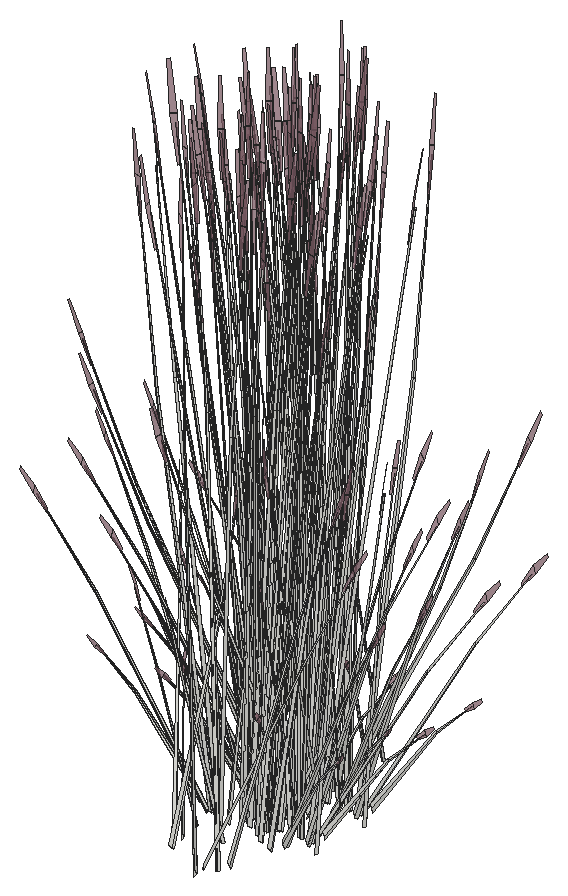
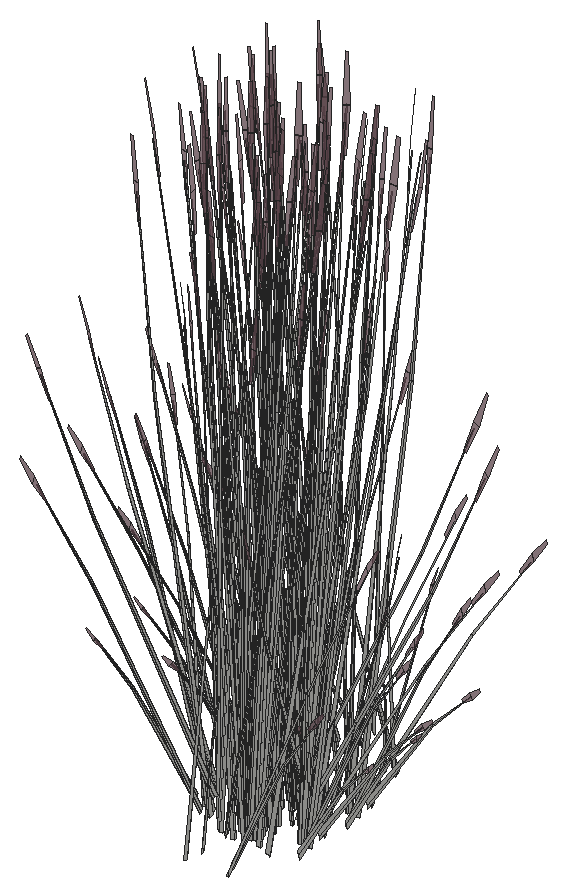
# SketchUp Ruby script. Lengths in inches.
U = 1.inch
M = Sketchup.active_model
def pt(a) = Geom::Point3d.new(a.map { |v| v * U })
def face(e, loops, mat)
  f = e.add_face(loops[0].map { |a| pt(a) })
  loops[1..].each { |l| e.add_face(l.map { |a| pt(a) }).erase! }
  f.material = f.back_material = mat if mat
  f
end
# faces: each face lists its corners as indices into pts; further lists are holes
def faces(e, pts, list, mat = nil) = list.each { |f| face(e, (f[0].is_a?(Array) ? f : [f]).map { |l| l.map { |i| pts[i] } }, mat) }
# xy, xz, yz: faces in a plane at the given z, y or x. An outline is a flat list of corners, or four numbers for a rectangle; further outlines are holes
def ring(l) = l.size == 4 ? [[l[0], l[1]], [l[2], l[1]], [l[2], l[3]], [l[0], l[3]]] : l.each_slice(2).to_a
def flat(e, list, mat, &to3) = list.each { |f| face(e, (f[0].is_a?(Array) ? f : [f]).map { |l| ring(l).map { |u, v| to3.(u, v) } }, mat) }
def xy(e, z, list, mat = nil) = flat(e, list, mat) { |x, y| [x, y, z] }
def xz(e, y, list, mat = nil) = flat(e, list, mat) { |x, z| [x, y, z] }
def yz(e, x, list, mat = nil) = flat(e, list, mat) { |y, z| [x, y, z] }
def lines(e, pts, list) = list.each { |a, b| e.add_line(pt(pts[a]), pt(pts[b])) }
# prism: a flat outline (further loops are holes) pulled along v
def prism(e, loops, v, mat = nil)
  f = face(e, loops, mat); d = Geom::Vector3d.new(v.map { |x| x * U })
  f.pushpull(f.normal.samedirection?(d) ? d.length : -d.length)
end
def box(e, o, s, mat = nil) = prism(e, [[o, [o[0] + s[0], o[1], o[2]], [o[0] + s[0], o[1] + s[1], o[2]], [o[0], o[1] + s[1], o[2]]]], [0, 0, s[2]], mat)
def at(x, y, z, deg = 0) = Geom::Transformation.translation(pt([x, y, z])) * Geom::Transformation.rotation(ORIGIN, Z_AXIS, deg.degrees)
def axes(o, x, y, z) = Geom::Transformation.new([*x, 0, *y, 0, *z, 0, *pt(o).to_a, 1])
def part(name) = M.definitions.add(name)
# library, detail: a bought-in or finely detailed component or shape, given as its bounding box
def library(name, o, s) = part(name).tap { |d| box(d.entities, o, s) }
def detail(e, o, s) = box(e.add_group.entities, o, s)
def put(e, d, t, mat = nil) = e.add_instance(d, t).tap { |i| i.material = mat if mat }
def group(e, t, mat = nil) = e.add_group.tap { |g| g.transformation = t; g.material = mat if mat }.entities
root = M.entities
M.materials.add("LightPink_Translucent").color = [144, 107, 117]
M.materials["LightPink_Translucent"].alpha = 0.75
c1 = part("blade")
p = [[2.15,0.21,22],[0,0.17,0],[0.09,0.45,0],[2.18,0.31,22],[2.29,0.31,22],[0.38,0.45,0],
  [2.48,0.24,33],[2.49,0.24,33],[2.48,0.22,33]]
faces(c1.entities,p,[[0,1,2,3],[4,5,2,3],[6,3,4,7],[8,0,3,6]])
c2 = part("seeds")
p = [[0.3,-0.1,1.38],[-0.01,-0.03,1.59],[-0.01,-0.03,0.03],[0.14,-0.07,-0.07],[0.29,-0.03,3],[0.15,0.01,3.11]]
faces(c2.entities,p,[[0,1,2,3],[1,0,4,5]],"LightPink_Translucent")
c3 = part("blade with seeds")
put(c3.entities,c1,at(0,0,0))
put(c3.entities,c2,axes([2.4,0.25,30.99],[1.5799,-0.05474,1.17369],[-0.12525,1.92788,0.29478],[-0.07173,-0.02425,1.56792]))
put(root,c3,axes([270.82,365.52,125.05],[-0.55932,-0.6538,0],[0.93577,-0.36461,-0.51607],[0.21313,-0.08304,1.63711]))
put(root,c3,axes([272.05,364.73,124.8],[-0.61821,0.37431,-0.03893],[-0.56645,-0.40995,-0.17649],[-0.03988,-0.11616,0.58215]))
put(root,c3,axes([274.52,360.68,125.02],[0.55932,0.6538,0],[-0.93577,0.36461,-0.51607],[-0.21313,0.08304,1.63711]))
put(root,c3,axes([274.04,358.09,125.49],[-0.02444,-0.61432,1.41272],[1.10603,0.15924,0.59816],[-0.26159,0.33615,1.3335]))
put(root,c3,axes([275.35,361.05,125.3125],[-0.57368,-0.02046,1.0506],[0.37886,-0.43461,0.58006],[0.22663,0.15441,0.8241]))
put(root,c3,axes([276.55,366.55,125.27],[-0.31959,-0.01933,1.43002],[-0.32741,-0.51843,-0.30754],[0.39262,-0.14666,0.61141]))
put(root,c3,axes([276.92,365.59,125.44],[-0.29798,0.33213,1.1486],[-0.25612,-0.44624,0.84392],[0.24611,-0.11182,0.25299]))
put(root,c3,axes([273.48,360,125.24],[0.01579,-0.21629,1.43002],[0.75442,-0.24159,-0.30754],[0.23289,0.25887,0.61141]))
put(root,c3,axes([268.98,365.41,124.8],[-0.25807,0.53277,-0.03893],[-0.79428,-0.16389,-0.17649],[-0.1206,-0.08714,0.58215]))
put(root,c3,axes([270.05,361.8,125.41],[-0.02315,-0.38796,1.1486],[0.57853,0.27671,0.84392],[-0.11378,0.18492,0.25299]))
put(root,c3,axes([268.55,367.84,125.05],[-1.11865,0,0],[0,-0.72922,-0.51607],[0,-0.16609,1.63711]))
put(root,c3,axes([268.74,366.54,125.27],[0.17466,0.18165,1.43002],[-0.40248,0.49377,-0.30754],[-0.41327,-0.11802,0.61141]))
put(root,c3,axes([269.57,360.97,125.47],[0.8127,-0.11554,0.06507],[0.18684,0.46549,-0.86304],[-0.05152,0.23564,0.7736]))
put(root,c3,axes([269.42,367.65,125.01],[-0.83213,0.54855,0.30756],[-0.83263,-0.54278,-0.36492],[-0.02906,-0.15578,1.64885]))
put(root,c3,axes([274.1,370.6,125.14],[-0.25429,0.13207,1.43002],[-0.76157,-0.23115,-0.30754],[0.14117,-0.28747,0.61141]))
put(root,c3,axes([272.94,371.0625,127.53],[-0.42698,-0.53052,-0.71045],[0.87893,-0.29566,0.08574],[-0.09984,-0.25633,1.00501]))
put(root,c3,axes([270.16,370.35,125.14],[-0.05417,0.21344,1.43002],[-0.79196,0.17867,-0.30754],[-0.18512,-0.27588,0.61141]))
put(root,c3,axes([272.0625,367.91,125.11],[1.00799,0.31623,0.24065],[-0.48511,0.65709,0.50002],[0,-0.15147,1.60543]))
put(root,c3,axes([271.67,368.8,125.11],[0.23711,-0.77313,-0.23429],[1.12425,0.13477,0.51271],[-0.19645,-0.10677,1.5644]))
put(root,c3,axes([267.7,367.09,125.44],[0.57115,-0.04669,1.1486],[-0.36229,0.41137,0.84392],[-0.28224,-0.06171,0.25299]))
put(root,c3,axes([274.72,371.58,127.53],[0.02328,-0.60353,-0.71045],[0.98022,0.04053,0.08574],[0.10344,-0.25568,1.00501]))
put(root,c3,axes([271.74,367.47,125.39],[-0.97146,0.04028,0.44739],[-0.08785,-0.66859,-0.21531],[0.17391,-0.06776,1.43643]))
put(root,c3,axes([269.23,367.96,125.15],[0,0.65246,0.49651],[-1.00089,0,0],[0,-0.1486,1.57504]))
put(root,c3,axes([269.38,361.46,125.24],[0.28231,-0.10293,1.43002],[0.69701,0.31035,-0.30754],[-0.20746,0.26854,0.61141]))
put(root,c3,axes([274.94,365.68,125.05],[0.55932,-0.6538,0],[0.93577,0.36461,-0.51607],[0.21313,0.08304,1.63711]))
put(root,c3,axes([271.7,367.71,125.04],[0.38895,0.72959,0.45755],[-1.11135,0.2537,0.17955],[0.01358,-0.13406,1.58856]))
put(root,c3,axes([273.16,369.55,125.3125],[0.11476,0.38047,1.1486],[-0.63664,-0.21072,0.84392],[0.06851,-0.19481,0.25299]))
put(root,c3,axes([277.14,368.27,124.66],[-0.57619,0.0783,1.41583],[-0.09171,-0.62326,0.08104],[0.40356,-0.09434,0.80566]))
put(root,c3,axes([278.19,367.72,124.9375],[-0.55463,-0.41721,-0.06488],[0.60744,-0.38228,-0.29416],[0.17212,-0.02691,0.97024]))
put(root,c3,axes([271.51,368.28,125.39],[-0.43405,0.58792,0.44739],[-0.90188,-0.28295,-0.21531],[0,-0.13553,1.43643]))
put(root,c3,axes([273.1,367.77,124.88],[0,-0.75495,0],[1.11865,0,0],[0,0,1.79456]))
put(root,c3,axes([274.46,366.03,125.15],[-0.83726,-0.32623,0.49651],[0.50045,-0.58498,0],[0.19069,0.0743,1.57504]))
put(root,c3,axes([272.57,367.29,125.04],[-0.74176,0.59212,0.45755],[-0.88124,-0.52269,0.17955],[0.17882,-0.05909,1.58856]))
put(root,c3,axes([273.38,368.36,124.97],[-0.83213,-0.56158,-0.06131],[0.83263,-0.56193,0],[-0.02906,-0.01961,1.75571]))
put(root,c3,axes([271.29,366.32,125.15],[-0.25843,0.64844,0.17642],[-0.9457,-0.1835,0.35086],[0.16336,-0.00316,1.60407]))
put(root,c3,axes([269.89,370.01,125.3125],[0.46666,0.22709,1.1486],[-0.67962,0.13651,0.84392],[-0.14541,-0.17452,0.25299]))
put(root,c3,axes([271.02,371.21,127.53],[-0.76283,-0.31537,-0.71045],[0.54213,-0.55263,0.08574],[-0.27638,-0.1883,1.00501]))
put(root,c3,axes([273.26,367.04,125.29],[0.17258,-0.58229,0.1448],[0.84319,0.10108,-0.41347],[0.15345,0.05979,1.26744]))
put(root,c3,axes([271.8,368.42,125.04],[1.13071,0.13747,0.45755],[-0.23011,0.77639,0.17955],[-0.16524,-0.07497,1.58856]))
put(root,c3,axes([272.9,367.19,125.39],[-0.53742,-0.54764,0.44739],[0.81403,-0.38564,-0.21531],[0.17391,0.06776,1.43643]))
put(root,c3,axes([271.19,369.66,125.15],[0.96132,-0.17317,0.17642],[0.23737,0.64447,0.35086],[-0.08574,-0.0939,1.60407]))
put(root,c3,axes([273.86,367.9375,124.88],[1.00089,0,0],[0,0.67548,0],[0,0,1.78407]))
put(root,c3,axes([274.15,366.36,125.15],[-0.96132,0.17317,0.17642],[-0.23737,-0.64447,0.35086],[0.08574,0.0939,1.60407]))
put(root,c3,axes([275.875,372.63,127.53],[0.4673,-0.51481,-0.71045],[0.81887,0.36587,0.08574],[0.27902,-0.18652,1.00501]))
put(root,c3,axes([273.54,367.6,125.06],[-1.13071,-0.13747,0.49198],[0.23011,-0.77639,0.19306],[0.16524,0.07497,1.70813]))
put(root,c3,axes([270.82,371.13,124.92],[-0.55932,-0.6538,0],[0.93577,-0.36461,-0.51607],[0.21313,-0.08304,1.63711]))
put(root,c3,axes([272.64,369.51,124.88],[-0.29189,-0.56252,0],[0.83351,-0.19699,0],[0,0,1.54371]))
put(root,c3,axes([272.05,370.35,124.68],[-0.61821,0.37431,-0.03893],[-0.56645,-0.40995,-0.17649],[-0.03988,-0.11616,0.58215]))
put(root,c3,axes([272.08,368.98,125.29],[-0.17258,0.58229,0.1448],[-0.84319,-0.10108,-0.41347],[-0.15345,-0.05979,1.26744]))
put(root,c3,axes([274.05,369.7,125.15],[0.25843,-0.64844,0.17642],[0.9457,0.1835,0.35086],[-0.16336,0.00316,1.60407]))
put(root,c3,axes([273.84,368.23,124.89],[0.62448,0.42144,0],[-0.62448,0.42144,0],[0,0,1.69266]))
put(root,c3,axes([275.53,368.05,125.15],[-0.70288,-0.47526,0.17642],[0.70832,-0.46097,0.35086],[-0.07763,0.09706,1.60407]))
put(root,c3,axes([278.34,368.48,125.44],[-0.55274,0.10771,1.1486],[0.26018,-0.44517,0.84392],[0.29323,0.03046,0.25299]))
put(root,c3,axes([272.43,369.77,124.87],[-0.90188,-0.29293,0],[0.43405,-0.60866,0],[0,0,1.62707]))
put(root,c3,axes([273.18,368.99,125.14],[-0.87356,-0.52515,-0.25192],[0.73507,-0.5897,0.5513],[-0.23523,0.06143,1.68216]))
put(root,c3,axes([270.88,369.99,125.15],[0.83726,0.32623,0.49651],[-0.50045,0.58498,0],[-0.19069,-0.0743,1.57504]))
put(root,c3,axes([276.55,372.16,125.14],[-0.31959,-0.01933,1.43002],[-0.32741,-0.51843,-0.30754],[0.39262,-0.14666,0.61141]))
put(root,c3,axes([273.83,367.74,125.39],[0.43405,-0.58792,0.44739],[0.90188,0.28295,-0.21531],[0,0.13553,1.43643]))
put(root,c3,axes([276.92,371.21,125.3125],[-0.29798,0.33213,1.1486],[-0.25612,-0.44624,0.84392],[0.24611,-0.11182,0.25299]))
put(root,c3,axes([273.67,368.07,124.97],[0,0.75458,-0.05637],[-1.11865,0,0],[0,0.02371,1.79368]))
put(root,c3,axes([270.4,370.33,125.05],[-0.55932,0.6538,0],[-0.93577,-0.36461,-0.51607],[-0.21313,-0.08304,1.63711]))
put(root,c3,axes([276.11,368.0625,125.15],[0,-0.65246,0.49651],[1.00089,0,0],[0,0.1486,1.57504]))
put(root,c3,axes([273.6,368.55,125.39],[0.97146,-0.04028,0.44739],[0.08785,0.66859,-0.21531],[-0.17391,0.06776,1.43643]))
put(root,c3,axes([274.21,367.87,125.29],[0.83351,-0.19028,0.1448],[0.29189,0.54335,-0.41347],[0,0.11958,1.26744]))
put(root,c3,axes([277.31,369.19,125.27],[-0.21545,-0.16047,1.43002],[0.28033,-0.53085,-0.30754],[0.43591,0.07191,0.61141]))
put(root,c3,axes([268.98,371.03,124.68],[-0.25807,0.53277,-0.03893],[-0.79428,-0.16389,-0.17649],[-0.1206,-0.08714,0.58215]))
put(root,c3,axes([268.55,373.46,124.92],[-1.11865,0,0],[0,-0.72922,-0.51607],[0,-0.16609,1.63711]))
put(root,c3,axes([273.45,369.78,124.88],[0.90188,0.29293,0],[-0.43405,0.60866,0],[0,0,1.74954]))
put(root,c3,axes([268.74,372.16,125.14],[0.17466,0.18165,1.43002],[-0.40248,0.49377,-0.30754],[-0.41327,-0.11802,0.61141]))
put(root,c3,axes([273.8125,370.43,124.87],[-0.55235,-0.65609,-0.05142],[0.93577,-0.36461,0.51607],[-0.23059,0.06247,1.6363]))
put(root,c3,axes([269.46,371.99,127.53],[-0.89428,-0.01571,-0.71045],[0.06006,-0.66153,0.08574],[-0.37886,-0.06981,1.00501]))
put(root,c3,axes([273.62,368.84,125.29],[0.66093,0.39201,0.1448],[-0.5513,0.44227,-0.41347],[-0.15345,0.05979,1.26744]))
put(root,c3,axes([274.32,370.05,125.15],[0.83726,-0.32623,0.49651],[0.50045,0.58498,0],[-0.19069,0.0743,1.57504]))
put(root,c3,axes([269.42,373.27,124.88],[-0.83213,0.54855,0.30756],[-0.83263,-0.54278,-0.36492],[-0.02906,-0.15578,1.64885]))
put(root,c3,axes([273.13,369.53,124.97],[0.38895,0.74956,-0.06012],[-1.11135,0.26265,0],[0.01358,0.02618,1.72173]))
put(root,c3,axes([267.54,369.19,125.27],[0.3109,0.05356,1.43002],[0.20038,0.54709,-0.30754],[-0.42231,0.10241,0.61141]))
put(root,c3,axes([276.79,368.17,125.05],[1.11865,0,0],[0,0.72922,-0.51607],[0,0.16609,1.63711]))
put(root,c3,axes([272.0625,373.52,124.98],[1.00799,0.31623,0.24065],[-0.48511,0.65709,0.50002],[0,-0.15147,1.60543]))
put(root,c3,axes([276.34,368.55,124.875],[-1.1181,-0.00522,-0.04976],[0,-0.72922,0.49943],[-0.03514,0.166,1.58352]))
put(root,c3,axes([266.89,370.34,125.44],[0.37283,-0.29571,1.1486],[0.14711,0.46813,0.84392],[-0.26943,0.08382,0.25299]))
put(root,c3,axes([267.7,372.7,125.3125],[0.57115,-0.04669,1.1486],[-0.36229,0.41137,0.84392],[-0.28224,-0.06171,0.25299]))
put(root,c3,axes([271.74,373.08,125.27],[-0.97146,0.04028,0.44739],[-0.08785,-0.66859,-0.21531],[0.17391,-0.06776,1.43643]))
put(root,c3,axes([269.23,373.57,125.03],[0,0.65246,0.49651],[-1.00089,0,0],[0,-0.1486,1.57504]))
put(root,c3,axes([274.94,371.3,124.92],[0.55932,-0.6538,0],[0.93577,0.36461,-0.51607],[0.21313,0.08304,1.63711]))
put(root,c3,axes([271.7,373.32,124.91],[0.38895,0.72959,0.45755],[-1.11135,0.2537,0.17955],[0.01358,-0.13406,1.58856]))
put(root,c3,axes([277.14,373.88,124.53],[-0.57619,0.0783,1.41583],[-0.09171,-0.62326,0.08104],[0.40356,-0.09434,0.80566]))
put(root,c3,axes([278.19,373.33,124.81],[-0.55463,-0.41721,-0.06488],[0.60744,-0.38228,-0.29416],[0.17212,-0.02691,0.97024]))
put(root,c3,axes([271.51,373.9,125.27],[-0.43405,0.58792,0.44739],[-0.90188,-0.28295,-0.21531],[0,-0.13553,1.43643]))
put(root,c3,axes([273.84,370.09,125.01],[1.11998,0.21207,0.30756],[-0.2802,0.75803,-0.36492],[-0.18537,0.09487,1.64885]))
put(root,c3,axes([273.1,373.38,124.75],[0,-0.75495,0],[1.11865,0,0],[0,0,1.79456]))
put(root,c3,axes([274.46,371.64,125.03],[-0.83726,-0.32623,0.49651],[0.50045,-0.58498,0],[0.19069,0.0743,1.57504]))
put(root,c3,axes([276.1,373.93,127.53],[0.78611,-0.28816,-0.71045],[0.4381,0.59317,0.08574],[0.37982,-0.06738,1.00501]))
put(root,c3,axes([272.57,372.91,124.91],[-0.74176,0.59212,0.45755],[-0.88124,-0.52269,0.17955],[0.17882,-0.05909,1.58856]))
put(root,c3,axes([275.27,370.02,125.44],[-0.5037,-0.18761,1.1486],[0.6504,-0.19062,0.84392],[0.17543,0.16147,0.25299]))
put(root,c3,axes([273.38,373.97,124.85],[-0.83213,-0.56158,-0.06131],[0.83263,-0.56193,0],[-0.02906,-0.01961,1.75571]))
put(root,c3,axes([271.29,371.93,125.02],[-0.25843,0.64844,0.17642],[-0.9457,-0.1835,0.35086],[0.16336,-0.00316,1.60407]))
put(root,c3,axes([273.26,372.65,125.16],[0.17258,-0.58229,0.1448],[0.84319,0.10108,-0.41347],[0.15345,0.05979,1.26744]))
put(root,c3,axes([274.52,370.5,125.05],[0.55932,0.6538,0],[-0.93577,0.36461,-0.51607],[-0.21313,0.08304,1.63711]))
put(root,c3,axes([271.8,374.04,124.91],[1.13071,0.13747,0.45755],[-0.23011,0.77639,0.17955],[-0.16524,-0.07497,1.58856]))
put(root,c3,axes([272.9,372.81,125.27],[-0.53742,-0.54764,0.44739],[0.81403,-0.38564,-0.21531],[0.17391,0.06776,1.43643]))
put(root,c3,axes([271.19,375.28,125.02],[0.96132,-0.17317,0.17642],[0.23737,0.64447,0.35086],[-0.08574,-0.0939,1.60407]))
put(root,c3,axes([275.35,370.875,125.34],[-0.57368,-0.02046,1.0506],[0.37886,-0.43461,0.58006],[0.22663,0.15441,0.8241]))
put(root,c3,axes([273.86,373.55,124.75],[1.00089,0,0],[0,0.67548,0],[0,0,1.78407]))
put(root,c3,axes([274.15,371.97,125.02],[-0.96132,0.17317,0.17642],[-0.23737,-0.64447,0.35086],[0.08574,0.0939,1.60407]))
put(root,c3,axes([273.48,369.82,125.27],[0.01579,-0.21629,1.43002],[0.75442,-0.24159,-0.30754],[0.23289,0.25887,0.61141]))
put(root,c3,axes([273.54,373.21,124.93],[-1.13071,-0.13747,0.49198],[0.23011,-0.77639,0.19306],[0.16524,0.07497,1.70813]))
put(root,c3,axes([272.64,375.125,124.75],[-0.29189,-0.56252,0],[0.83351,-0.19699,0],[0,0,1.54371]))
put(root,c3,axes([272.08,374.59,125.16],[-0.17258,0.58229,0.1448],[-0.84319,-0.10108,-0.41347],[-0.15345,-0.05979,1.26744]))
put(root,c3,axes([270.05,371.625,125.44],[-0.02315,-0.38796,1.1486],[0.57853,0.27671,0.84392],[-0.11378,0.18492,0.25299]))
put(root,c3,axes([274.05,375.3125,125.02],[0.25843,-0.64844,0.17642],[0.9457,0.1835,0.35086],[-0.16336,0.00316,1.60407]))
put(root,c3,axes([273.84,373.84,124.76],[0.62448,0.42144,0],[-0.62448,0.42144,0],[0,0,1.69266]))
put(root,c3,axes([275.53,373.66,125.02],[-0.70288,-0.47526,0.17642],[0.70832,-0.46097,0.35086],[-0.07763,0.09706,1.60407]))
put(root,c3,axes([278.34,374.09,125.3125],[-0.55274,0.10771,1.1486],[0.26018,-0.44517,0.84392],[0.29323,0.03046,0.25299]))
put(root,c3,axes([272.43,375.38,124.74],[-0.90188,-0.29293,0],[0.43405,-0.60866,0],[0,0,1.62707]))
put(root,c3,axes([270.88,375.61,125.03],[0.83726,0.32623,0.49651],[-0.50045,0.58498,0],[-0.19069,-0.0743,1.57504]))
put(root,c3,axes([269.57,370.79,125.5],[0.8127,-0.11554,0.06507],[0.18684,0.46549,-0.86304],[-0.05152,0.23564,0.7736]))
put(root,c3,axes([273.83,373.35,125.27],[0.43405,-0.58792,0.44739],[0.90188,0.28295,-0.21531],[0,0.13553,1.43643]))
put(root,c3,axes([273.67,373.69,124.84],[0,0.75458,-0.05637],[-1.11865,0,0],[0,0.02371,1.79368]))
put(root,c3,axes([270.4,375.95,124.92],[-0.55932,0.6538,0],[-0.93577,-0.36461,-0.51607],[-0.21313,-0.08304,1.63711]))
put(root,c3,axes([276.11,373.68,125.03],[0,-0.65246,0.49651],[1.00089,0,0],[0,0.1486,1.57504]))
put(root,c3,axes([273.6,374.16,125.27],[0.97146,-0.04028,0.44739],[0.08785,0.66859,-0.21531],[-0.17391,0.06776,1.43643]))
put(root,c3,axes([274.21,373.48,125.16],[0.83351,-0.19028,0.1448],[0.29189,0.54335,-0.41347],[0,0.11958,1.26744]))
put(root,c3,axes([277.31,374.81,125.14],[-0.21545,-0.16047,1.43002],[0.28033,-0.53085,-0.30754],[0.43591,0.07191,0.61141]))
put(root,c3,axes([274.1,380.97,125.17],[-0.25429,0.13207,1.43002],[-0.76157,-0.23115,-0.30754],[0.14117,-0.28747,0.61141]))
put(root,c3,axes([273.45,375.39,124.75],[0.90188,0.29293,0],[-0.43405,0.60866,0],[0,0,1.74954]))
put(root,c3,axes([269.38,371.28,125.27],[0.28231,-0.10293,1.43002],[0.69701,0.31035,-0.30754],[-0.20746,0.26854,0.61141]))
put(root,c3,axes([270.16,380.72,125.17],[-0.05417,0.21344,1.43002],[-0.79196,0.17867,-0.30754],[-0.18512,-0.27588,0.61141]))
put(root,c3,axes([273.8125,376.04,124.74],[-0.55235,-0.65609,-0.05142],[0.93577,-0.36461,0.51607],[-0.23059,0.06247,1.6363]))
put(root,c3,axes([273.62,374.45,125.16],[0.66093,0.39201,0.1448],[-0.5513,0.44227,-0.41347],[-0.15345,0.05979,1.26744]))
put(root,c3,axes([275.33,375.13,127.53],[0.89428,0.01571,-0.71045],[-0.06006,0.66153,0.08574],[0.37886,0.06981,1.00501]))
put(root,c3,axes([274.32,375.66,125.03],[0.83726,-0.32623,0.49651],[0.50045,0.58498,0],[-0.19069,0.0743,1.57504]))
put(root,c3,axes([273.13,375.15,124.84],[0.38895,0.74956,-0.06012],[-1.11135,0.26265,0],[0.01358,0.02618,1.72173]))
put(root,c3,axes([267.54,374.8,125.14],[0.3109,0.05356,1.43002],[0.20038,0.54709,-0.30754],[-0.42231,0.10241,0.61141]))
put(root,c3,axes([273.16,379.92,125.35],[0.11476,0.38047,1.1486],[-0.63664,-0.21072,0.84392],[0.06851,-0.19481,0.25299]))
put(root,c3,axes([276.79,373.79,124.92],[1.11865,0,0],[0,0.72922,-0.51607],[0,0.16609,1.63711]))
put(root,c3,axes([276.34,374.16,124.75],[-1.1181,-0.00522,-0.04976],[0,-0.72922,0.49943],[-0.03514,0.166,1.58352]))
put(root,c3,axes([266.89,375.95,125.3125],[0.37283,-0.29571,1.1486],[0.14711,0.46813,0.84392],[-0.26943,0.08382,0.25299]))
put(root,c3,axes([269.89,380.37,125.35],[0.46666,0.22709,1.1486],[-0.67962,0.13651,0.84392],[-0.14541,-0.17452,0.25299]))
